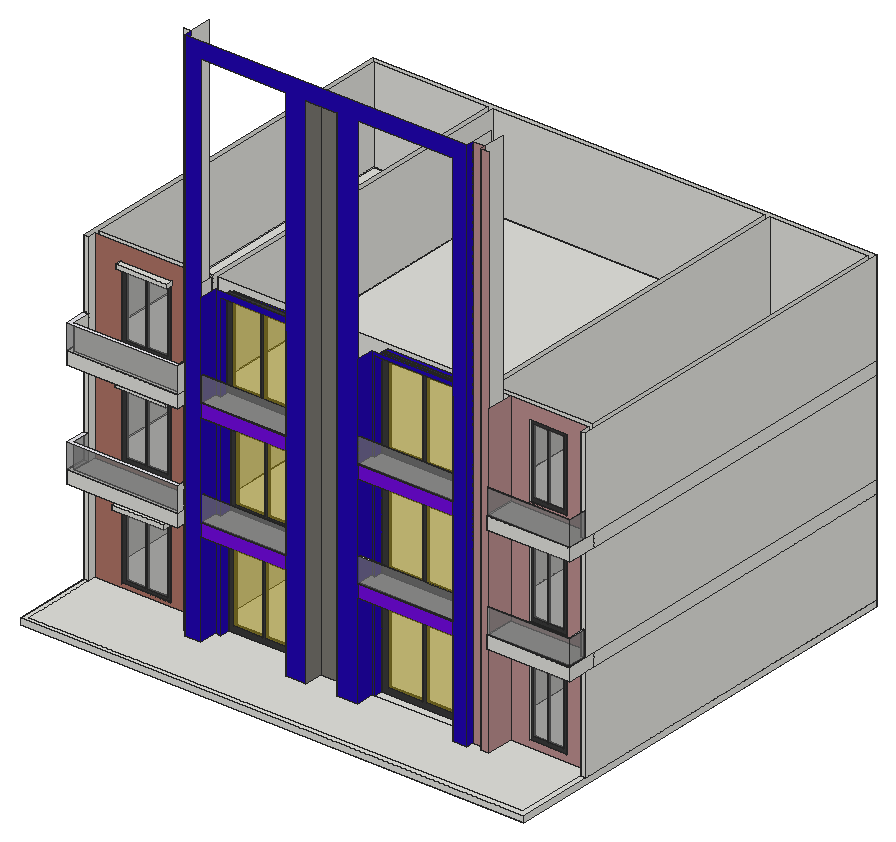
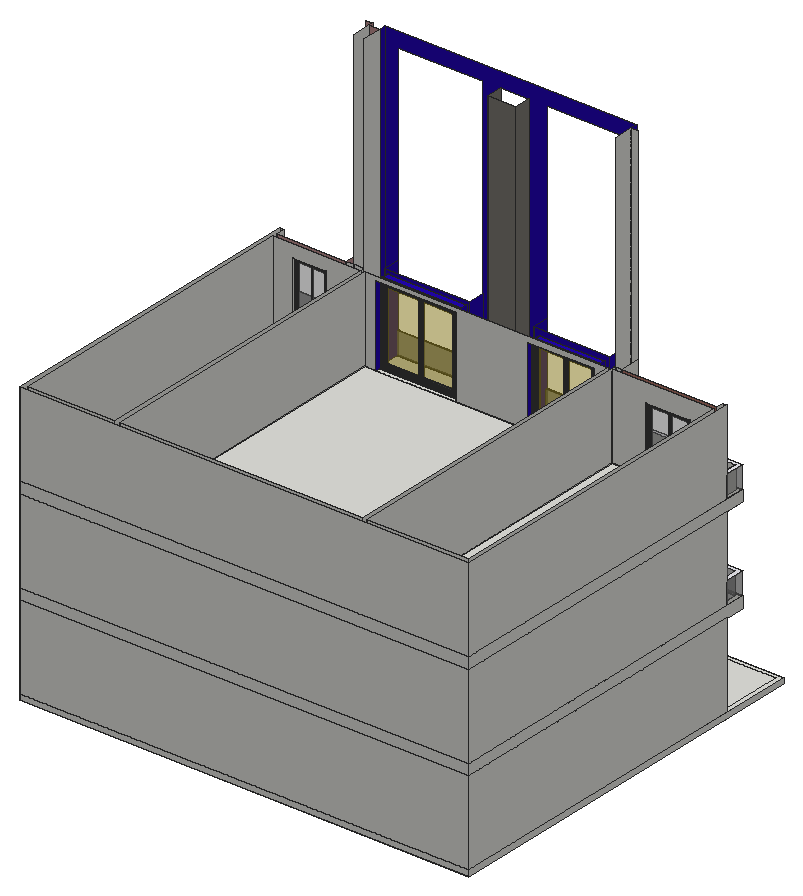
# SketchUp Ruby script. Lengths in inches.
U = 1.inch
M = Sketchup.active_model
def pt(a) = Geom::Point3d.new(a.map { |v| v * U })
def face(e, loops, mat)
  f = e.add_face(loops[0].map { |a| pt(a) })
  loops[1..].each { |l| e.add_face(l.map { |a| pt(a) }).erase! }
  f.material = f.back_material = mat if mat
  f
end
# faces: each face lists its corners as indices into pts; further lists are holes
def faces(e, pts, list, mat = nil) = list.each { |f| face(e, (f[0].is_a?(Array) ? f : [f]).map { |l| l.map { |i| pts[i] } }, mat) }
# xy, xz, yz: faces in a plane at the given z, y or x. An outline is a flat list of corners, or four numbers for a rectangle; further outlines are holes
def ring(l) = l.size == 4 ? [[l[0], l[1]], [l[2], l[1]], [l[2], l[3]], [l[0], l[3]]] : l.each_slice(2).to_a
def flat(e, list, mat, &to3) = list.each { |f| face(e, (f[0].is_a?(Array) ? f : [f]).map { |l| ring(l).map { |u, v| to3.(u, v) } }, mat) }
def xy(e, z, list, mat = nil) = flat(e, list, mat) { |x, y| [x, y, z] }
def xz(e, y, list, mat = nil) = flat(e, list, mat) { |x, z| [x, y, z] }
def yz(e, x, list, mat = nil) = flat(e, list, mat) { |y, z| [x, y, z] }
def lines(e, pts, list) = list.each { |a, b| e.add_line(pt(pts[a]), pt(pts[b])) }
# prism: a flat outline (further loops are holes) pulled along v
def prism(e, loops, v, mat = nil)
  f = face(e, loops, mat); d = Geom::Vector3d.new(v.map { |x| x * U })
  f.pushpull(f.normal.samedirection?(d) ? d.length : -d.length)
end
def box(e, o, s, mat = nil) = prism(e, [[o, [o[0] + s[0], o[1], o[2]], [o[0] + s[0], o[1] + s[1], o[2]], [o[0], o[1] + s[1], o[2]]]], [0, 0, s[2]], mat)
def at(x, y, z, deg = 0) = Geom::Transformation.translation(pt([x, y, z])) * Geom::Transformation.rotation(ORIGIN, Z_AXIS, deg.degrees)
def axes(o, x, y, z) = Geom::Transformation.new([*x, 0, *y, 0, *z, 0, *pt(o).to_a, 1])
def part(name) = M.definitions.add(name)
# library, detail: a bought-in or finely detailed component or shape, given as its bounding box
def library(name, o, s) = part(name).tap { |d| box(d.entities, o, s) }
def detail(e, o, s) = box(e.add_group.entities, o, s)
def put(e, d, t, mat = nil) = e.add_instance(d, t).tap { |i| i.material = mat if mat }
def group(e, t, mat = nil) = e.add_group.tap { |g| g.transformation = t; g.material = mat if mat }.entities
root = M.entities
M.materials.add("[0119_RosyBrown]").color = [188, 143, 143]
M.materials.add("[Brick Colored Blue]").color = [34, 5, 180]
M.materials.add("[Brick Colored Blue]1").color = [115, 11, 225]
M.materials.add("[Color M07]").color = [58, 58, 58]
M.materials.add("[Metal Silver]").color = [234, 233, 238]
M.materials.add("[Rough Square Concrete Block]").color = [123, 120, 113]
M.materials.add("[Stone Flagstone Ashlar]").color = [175, 116, 102]
M.materials.add("[Translucent Glass Blue]").color = [202, 178, 24]
M.materials["[Translucent Glass Blue]"].alpha = 0.5
M.materials.add("[Translucent Glass Gray]").color = [128, 128, 128]
M.materials["[Translucent Glass Gray]"].alpha = 0.5
c1 = part("Group\#2")
xy(c1.entities,0,[[0,0,124.375,6.5]],"[Color M07]")
xy(c1.entities,9.35,[[9.35,0,58.13,6.5],[62.66,0,115.02,6.5]],"[Color M07]")
xy(c1.entities,131.58,[[9.35,0,58.13,6.5],[62.66,0,115.02,6.5]],"[Color M07]")
xy(c1.entities,140.9375,[[0,0,124.375,6.5]],"[Color M07]")
xz(c1.entities,0,[[[0,0,124.375,140.9375],[62.66,9.35,115.02,131.58],[9.35,9.35,58.13,131.58]]],"[Color M07]")
xz(c1.entities,0,[[9.35,9.35,58.13,131.58],[62.66,9.35,115.02,131.58]],"[Translucent Glass Blue]")
xz(c1.entities,6.5,[[[0,0,124.375,140.9375],[62.66,9.35,115.02,131.58],[9.35,9.35,58.13,131.58]]],"[Color M07]")
yz(c1.entities,0,[[0,0,6.5,140.9375]],"[Color M07]")
yz(c1.entities,9.35,[[0,9.35,6.5,131.58]],"[Color M07]")
yz(c1.entities,58.13,[[0,9.35,6.5,131.58]],"[Color M07]")
yz(c1.entities,62.66,[[0,9.35,6.5,131.58]],"[Color M07]")
yz(c1.entities,115.02,[[0,9.35,6.5,131.58]],"[Color M07]")
yz(c1.entities,124.375,[[0,0,6.5,140.9375]],"[Color M07]")
c2 = part("Group\#1")
xy(c2.entities,0,[[0,0,103.0625,5.375]],"[Color M07]")
xy(c2.entities,8.61,[[8.61,0,48.54,5.375],[51.97,0,94.45,5.375]],"[Color M07]")
xy(c2.entities,158.15,[[8.61,0,48.54,5.375],[51.97,0,94.45,5.375]],"[Color M07]")
xy(c2.entities,166.76,[[0,0,103.0625,5.375]],"[Color M07]")
xz(c2.entities,0,[[[0,0,103.0625,166.76],[51.97,8.61,94.45,158.15],[8.61,8.61,48.54,158.15]]],"[Color M07]")
xz(c2.entities,0,[[8.61,8.61,48.54,158.15],[51.97,8.61,94.45,158.15]],"[Translucent Glass Gray]")
xz(c2.entities,5.375,[[[0,0,103.0625,166.76],[51.97,8.61,94.45,158.15],[8.61,8.61,48.54,158.15]]],"[Color M07]")
yz(c2.entities,0,[[0,0,5.375,166.76]],"[Color M07]")
yz(c2.entities,8.61,[[0,8.61,5.375,158.15]],"[Color M07]")
yz(c2.entities,48.54,[[0,8.61,5.375,158.15]],"[Color M07]")
yz(c2.entities,51.97,[[0,8.61,5.375,158.15]],"[Color M07]")
yz(c2.entities,94.45,[[0,8.61,5.375,158.15]],"[Color M07]")
yz(c2.entities,103.0625,[[0,0,5.375,166.76]],"[Color M07]")
xy(root,0,[[0,0,960,840]])
xy(root,12,[[0,0,960,0,960,147.0625,951,147.0625,951,9,9,9,9,151.625,0,151.625],[9,9,951,9,951,166.4375,801.6875,166.4375,801.6875,115.3125,786.375,115.3125,786.375,124.625,763.625,124.625,763.625,110.3125,736.375,110.3125,736.375,145,554.39,145,554.39,110.3125,515.65,110.3125,515.65,145,456.7,145,456.7,110.3125,417.96,110.3125,417.96,145,405.4,145,405.4,175.4375,265.83,175.4375,265.83,145,255.8125,145,255.8125,110.3125,226.3125,110.3125,226.3125,124.375,212.1875,124.375,212.1875,166.4375,9,166.4375],[[226.3125,110.3125,226.3125,166.4375,9,166.4375,9,151.625,0,151.625,0,840,960,840,960,147.0625,951,147.0625,951,166.4375,763.625,166.4375,763.625,110.3125,736.375,110.3125,736.375,145,730.3125,145,730.3125,175.4375,754.625,175.4375,754.625,831,235.3125,831,235.3125,175.4375,265.83,175.4375,265.83,145,255.8125,145,255.8125,110.3125],[9,175.4375,226.3125,831],[763.625,175.4375,951,831]],[417.96,110.3125,417.96,145,405.4,145,405.4,175.4375,560.75,175.4375,560.75,145,554.39,145,554.39,110.3125,515.65,110.3125,515.65,145,456.7,145,456.7,110.3125],[786.375,115.3125,801.6875,166.4375],
  [212.1875,124.375,226.3125,166.4375],[763.625,124.625,786.375,166.4375],[560.75,145,730.3125,175.4375],[9,175.4375,226.3125,831],[235.3125,175.4375,754.625,831],
  [763.625,175.4375,951,831]])
xy(root,19.77,[[59.43,166.4375,154.62,175.4375]])
xy(root,24.53,[[838.25,166.4375,907.94,175.4375]])
xy(root,152.51,[[57.84,146.25,57.84,166.4375,59.43,166.4375,59.43,175.4375,154.62,175.4375,154.62,166.4375,155.9,166.4375,155.9,146.25]])
xy(root,162.04,[[57.84,146.25,155.9,166.4375]])
xy(root,164.9,[[838.25,166.4375,907.94,175.4375]])
xy(root,178.5,[[265.83,145,405.4,175.4375]],"[Brick Colored Blue]")
xy(root,184.85,[[560.75,145,730.3125,175.4375]],"[Brick Colored Blue]")
xy(root,192,[[0,110.3125,9,151.625],[9,110.3125,212.1875,166.4375],[255.8125,110.3125,417.96,145],[554.39,110.3125,736.375,145],[801.6875,110.3125,801.6875,166.4375,951,166.4375,951,147.0625,960,147.0625,960,110.3125]])
xy(root,210,[[9,175.4375,226.3125,831],[235.3125,175.4375,754.625,831]])
xy(root,213,[[763.625,175.4375,951,831]])
xy(root,216,[[0,110.3125,0,151.625,9,151.625,9,117.34,210.0625,117.34,210.0625,124.375,212.1875,124.375,212.1875,110.3125],[255.8125,110.3125,417.96,111.6875],[554.39,110.3125,736.375,111.6875],[801.6875,110.3125,960,110.3125,960,147.0625,959.125,147.0625,959.125,110.8125,801.6875,110.8125],[801.6875,110.8125,802.5,115.3125],
  [802.5,110.8125,802.5,113,956.625,113,956.625,147.0625,959.125,147.0625,959.125,110.8125],[255.8125,111.6875,417.96,113.6875],[554.39,111.6875,736.375,113.6875],[802.5,113,956.625,113,956.625,147.0625,951,147.0625,951,166.4375,801.6875,166.4375,801.6875,115.3125,802.5,115.3125],[255.8125,113.6875,417.96,113.6875,417.96,145,405.4,145,405.4,175.4375,265.83,175.4375,265.83,145,255.8125,145],
  [554.39,113.6875,736.375,113.6875,736.375,145,730.3125,145,730.3125,175.4375,560.75,175.4375,560.75,145,554.39,145],[9,117.34,210.0625,117.34,210.0625,124.375,212.1875,124.375,212.1875,166.4375,9,166.4375],[9,175.4375,226.3125,831],[235.3125,175.4375,754.625,831],[763.625,175.4375,951,831]])
xy(root,226.89,[[59.43,166.4375,154.62,175.4375]])
xy(root,227.09,[[838.25,166.4375,907.94,175.4375]])
xy(root,264,[[0,110.3125,212.1875,110.3125,212.1875,124.375,210.0625,124.375,210.0625,117.34,9,117.34,9,151.625,0,151.625],[802.5,110.8125,959.125,110.8125,959.125,147.0625,956.625,147.0625,956.625,113,802.5,113],[255.8125,111.6875,417.96,113.6875],[554.39,111.6875,736.375,113.6875]],"[Metal Silver]")
xy(root,359.63,[[57.84,152.125,57.84,166.4375,59.43,166.4375,59.43,175.4375,154.62,175.4375,154.62,166.4375,155.9,166.4375,155.9,152.125]])
xy(root,367.47,[[838.25,166.4375,907.94,175.4375]])
xy(root,368.04,[[57.84,152.125,155.9,166.4375]])
xy(root,382.81,[[265.83,145,405.4,175.4375]],"[Brick Colored Blue]")
xy(root,387.91,[[560.75,145,730.3125,175.4375]])
xy(root,396,[[0,110.3125,9,151.625],[9,110.3125,212.1875,166.4375],[255.8125,110.3125,417.96,145],[554.39,110.3125,736.375,145],[801.6875,110.3125,801.6875,166.4375,951,166.4375,951,147.0625,960,147.0625,960,110.3125]])
xy(root,409.875,[[763.625,175.4375,951,831]])
xy(root,414,[[9,175.4375,226.3125,831],[235.3125,175.4375,754.625,831]])
xy(root,420,[[0,110.3125,0,151.625,9,151.625,9,117.34,208.125,117.34,208.125,124.375,212.1875,124.375,212.1875,110.3125],[255.8125,110.3125,417.96,111.8125],[554.39,110.3125,736.375,111.8125],[801.6875,110.3125,960,110.3125,960,147.0625,959.6875,147.0625,959.6875,110.8125,801.6875,110.8125],[801.6875,110.8125,802.125,115.3125],
  [802.125,110.8125,802.125,111.5625,958.9375,111.5625,958.9375,147.0625,959.6875,147.0625,959.6875,110.8125],[802.125,111.5625,958.9375,111.5625,958.9375,147.0625,951,147.0625,951,166.4375,801.6875,166.4375,801.6875,115.3125,802.125,115.3125],[255.8125,111.8125,417.96,113.8125],[554.39,111.8125,736.375,113.8125],[255.8125,113.8125,417.96,113.8125,417.96,145,405.4,145,405.4,175.4375,265.83,175.4375,265.83,145,255.8125,145],
  [554.39,113.8125,736.375,113.8125,736.375,145,730.3125,145,730.3125,175.4375,560.75,175.4375,560.75,145,554.39,145],[9,117.34,208.125,117.34,208.125,124.375,212.1875,124.375,212.1875,166.4375,9,166.4375],[9,175.4375,226.3125,831],[235.3125,175.4375,754.625,831],[763.625,175.4375,951,831]])
xy(root,428.14,[[59.43,166.4375,154.62,175.4375]])
xy(root,432.47,[[838.25,166.4375,907.94,175.4375]])
xy(root,468,[[802.125,110.8125,959.6875,110.8125,959.6875,147.0625,958.9375,147.0625,958.9375,111.5625,802.125,111.5625]])
xy(root,468,[[255.8125,111.8125,417.96,113.8125],[554.39,111.8125,736.375,113.8125]],"[Metal Silver]")
xy(root,468.3125,[[0,110.3125,212.1875,110.3125,212.1875,124.375,208.125,124.375,208.125,117.34,9,117.34,9,151.625,0,151.625]],"[Metal Silver]")
xy(root,560.88,[[57.84,154.25,57.84,166.4375,59.43,166.4375,59.43,175.4375,154.62,175.4375,154.62,166.4375,155.9,166.4375,155.9,154.25]])
xy(root,568.66,[[57.84,154.25,155.9,166.4375]])
xy(root,572.84,[[838.25,166.4375,907.94,175.4375]])
xy(root,587.81,[[265.83,145,405.4,175.4375]],"[Brick Colored Blue]")
xy(root,592.22,[[560.75,145,730.3125,175.4375]],"[Brick Colored Blue]")
xz(root,0,[[0,0,960,12]])
xz(root,110.3125,[[0,192,212.1875,216],[801.6875,192,960,216],[0,396,212.1875,420],[801.6875,396,960,420]])
xz(root,110.3125,[[226.3125,12,255.8125,12,255.8125,1008,417.96,1008,417.96,12,456.7,12,456.7,1008,515.65,1008,515.65,12,554.39,12,554.39,1008,736.375,1008,736.375,12,763.625,12,763.625,1039.1875,226.3125,1039.1875]],"[Brick Colored Blue]")
xz(root,110.3125,[[255.8125,192,417.96,216],[554.39,192,736.375,216],[255.8125,396,417.96,420],[554.39,396,736.375,420]],"[Brick Colored Blue]1")
xz(root,110.3125,[[0,216,212.1875,264],[0,420,212.1875,468.3125]],"[Translucent Glass Gray]")
xz(root,110.8125,[[802.5,216,959.125,264],[802.125,420,959.6875,468]],"[Translucent Glass Gray]")
xz(root,111.5625,[[802.125,420,958.9375,468]],"[Translucent Glass Gray]")
xz(root,111.6875,[[255.8125,216,417.96,264],[554.39,216,736.375,264]],"[Translucent Glass Gray]")
xz(root,111.8125,[[255.8125,420,417.96,468],[554.39,420,736.375,468]],"[Translucent Glass Gray]")
xz(root,113,[[802.5,216,956.625,264]],"[Translucent Glass Gray]")
xz(root,113.6875,[[255.8125,216,417.96,264],[554.39,216,736.375,264]],"[Translucent Glass Gray]")
xz(root,113.8125,[[255.8125,420,417.96,468],[554.39,420,736.375,468]],"[Translucent Glass Gray]")
xz(root,115.3125,[[786.375,12,801.6875,1039.1875]],"[0119_RosyBrown]")
xz(root,117.34,[[9,420,208.125,468.3125]])
xz(root,117.34,[[9,216,210.0625,264]],"[Translucent Glass Gray]")
xz(root,124.375,[[212.1875,12,226.3125,1039.1875],[210.0625,216,212.1875,264],[208.125,420,212.1875,468.3125],[226.3125,420,229.5,600]])
xz(root,124.625,[[763.625,12,786.375,1039.1875]],"[0119_RosyBrown]")
xz(root,145,[[255.8125,12,265.83,12,265.83,178.5,405.4,178.5,405.4,12,417.96,12,417.96,192,255.8125,192],[554.39,12,560.75,12,560.75,184.85,730.3125,184.85,730.3125,12,736.375,12,736.375,192,554.39,192],[255.8125,216,265.83,216,265.83,382.81,405.4,382.81,405.4,216,417.96,216,417.96,396,255.8125,396],[554.39,216,560.75,216,560.75,387.91,730.3125,387.91,730.3125,216,736.375,216,736.375,396,554.39,396],[255.8125,420,265.83,420,265.83,587.81,405.4,587.81,405.4,420,417.96,420,417.96,600,255.8125,600],
  [554.39,420,560.75,420,560.75,592.22,730.3125,592.22,730.3125,420,736.375,420,736.375,600,554.39,600]],"[Brick Colored Blue]")
xz(root,145,[[456.7,12,515.65,1008]],"[Rough Square Concrete Block]")
xz(root,146.25,[[57.84,152.51,155.9,162.04]])
xz(root,147.0625,[[951,12,960,192],[951,216,956.625,216,956.625,264,959.125,264,959.125,216,960,216,960,396,951,396],[956.625,216,959.125,264],[951,420,958.9375,420,958.9375,468,959.6875,468,959.6875,420,960,420,960,600,951,600],[958.9375,420,959.6875,468]])
xz(root,151.625,[[2.39,-3.36,6.71,0.95],[2.39,5.08,6.71,9.39],[0,12,9,192],[2.38,209.32,6.44,213.38],[0,216,9,264],
  [0,264,9,396],[2.1,413.18,6.41,417.5],[0,420,9,468],[0,468,9,468.3125],[0,468.3125,9,600]])
xz(root,152.125,[[57.84,359.63,155.9,368.04]])
xz(root,154.25,[[57.84,560.88,155.9,568.66]])
xz(root,166.4375,[[212.1875,12,226.3125,192],[763.625,12,786.375,192],[786.375,12,801.6875,192],[217.1875,192,226.3125,216],[763.625,192,786.375,216],
  [786.375,192,801.6875,216],[212.1875,216,226.3125,396],[763.625,216,786.375,396],[786.375,216,801.6875,396],[217.1875,396,226.3125,420],
  [763.625,396,786.375,420],[786.375,396,801.6875,420],[212.1875,420,226.3125,600],[226.3125,420,229.5,600],[763.625,420,786.375,600],
  [786.375,420,801.6875,600]])
xz(root,166.4375,[[[801.6875,12,951,192],[838.25,24.53,907.94,164.9]],[[801.6875,216,951,396],[838.25,227.09,907.94,367.47]],[[801.6875,420,951,600],[838.25,432.47,907.94,572.84]]],"[0119_RosyBrown]")
xz(root,166.4375,[[[9,12,212.1875,192],[59.43,19.77,59.43,152.51,57.84,152.51,57.84,162.04,155.9,162.04,155.9,152.51,154.62,152.51,154.62,19.77]],[[9,216,212.1875,396],[59.43,226.89,59.43,359.63,57.84,359.63,57.84,368.04,155.9,368.04,155.9,359.63,154.62,359.63,154.62,226.89]],[[9,420,212.1875,600],[59.43,428.14,59.43,560.88,57.84,560.88,57.84,568.66,155.9,568.66,155.9,560.88,154.62,560.88,154.62,428.14]]],"[Stone Flagstone Ashlar]")
xz(root,175.4375,[[[9,12,226.3125,192],[59.43,19.77,154.62,152.51]],[235.3125,12,235.3125,192,754.625,192,754.625,12,730.3125,12,730.3125,184.85,560.75,184.85,560.75,12,405.4,12,405.4,178.5,265.83,178.5,265.83,12],[[763.625,12,951,192],[838.25,24.53,907.94,164.9]],[9,192,226.3125,210],[235.3125,192,754.625,210],
  [763.625,192,951,213],[9,210,226.3125,216],[235.3125,210,265.83,216],[265.83,210,405.4,216],[405.4,210,560.75,216],
  [560.75,210,730.3125,216],[730.3125,210,754.625,216],[763.625,213,951,216],[[9,216,226.3125,396],[59.43,226.89,154.62,359.63]],[235.3125,216,235.3125,396,754.625,396,754.625,216,730.3125,216,730.3125,387.91,560.75,387.91,560.75,216,405.4,216,405.4,382.81,265.83,382.81,265.83,216],
  [[763.625,216,951,396],[838.25,227.09,907.94,367.47]],[9,396,226.3125,414],[235.3125,396,754.625,414],[763.625,396,951,409.875],[763.625,409.875,951,420],
  [9,414,226.3125,420],[235.3125,414,265.83,420],[265.83,414,405.4,420],[405.4,414,560.75,420],[560.75,414,730.3125,420],
  [730.3125,414,754.625,420],[[9,420,226.3125,600],[59.43,428.14,154.62,560.88]],[235.3125,420,235.3125,600,754.625,600,754.625,420,730.3125,420,730.3125,592.22,560.75,592.22,560.75,420,405.4,420,405.4,587.81,265.83,587.81,265.83,420],[[763.625,420,951,600],[838.25,432.47,907.94,572.84]]])
xz(root,831,[[9,12,226.3125,192],[235.3125,12,754.625,192],[763.625,12,951,192],[9,192,226.3125,210],[235.3125,192,754.625,210],
  [763.625,192,951,213],[9,210,226.3125,216],[235.3125,210,754.625,216],[763.625,213,951,216],[9,216,226.3125,396],
  [235.3125,216,754.625,396],[763.625,216,951,396],[9,396,226.3125,414],[235.3125,396,754.625,414],[763.625,396,951,409.875],
  [763.625,409.875,951,420],[9,414,226.3125,420],[235.3125,414,754.625,420],[9,420,226.3125,600],[235.3125,420,754.625,600],
  [763.625,420,951,600]])
xz(root,840,[[0,0,960,12],[0,12,960,192],[0,192,960,216],[0,216,960,396],[0,396,960,420],
  [0,420,960,600]])
yz(root,0,[[0,0,840,12],[151.625,12,840,192],[110.3125,192,840,216],[151.625,216,840,396],[110.3125,396,840,420],
  [151.625,420,840,600]])
yz(root,0,[[110.3125,216,151.625,264],[110.3125,420,151.625,468.3125]],"[Translucent Glass Gray]")
yz(root,9,[[151.625,12,166.4375,192],[175.4375,12,831,192],[175.4375,192,831,210],[175.4375,210,200.26,216],[200.26,210,214.57,216],
  [214.57,210,831,216],[151.625,216,166.4375,396],[175.4375,216,831,396],[175.4375,396,831,414],[175.4375,414,236.35,420],
  [236.35,414,248.35,420],[248.35,414,831,420],[117.34,420,151.625,468.3125],[151.625,420,166.4375,600],[175.4375,420,831,600]])
yz(root,9,[[117.34,216,151.625,264]],"[Translucent Glass Gray]")
yz(root,57.84,[[146.25,152.51,166.4375,162.04],[152.125,359.63,166.4375,368.04],[154.25,560.88,166.4375,568.66]])
yz(root,59.43,[[166.4375,19.77,175.4375,152.51],[166.4375,226.89,175.4375,359.63],[166.4375,428.14,175.4375,560.88]])
yz(root,154.62,[[166.4375,19.77,175.4375,152.51],[166.4375,226.89,175.4375,359.63],[166.4375,428.14,175.4375,560.88]])
yz(root,155.9,[[146.25,152.51,166.4375,162.04],[152.125,359.63,166.4375,368.04],[154.25,560.88,166.4375,568.66]])
yz(root,208.125,[[117.34,420,124.375,468.3125]])
yz(root,210.0625,[[117.34,216,124.375,264]])
yz(root,212.1875,[[124.375,12,166.4375,192],[110.3125,192,124.375,216],[110.3125,216,124.375,264],[124.375,216,166.4375,396],[110.3125,396,124.375,420],
  [110.3125,420,124.375,468.3125],[124.375,420,166.4375,600]])
yz(root,226.3125,[[124.375,12,166.4375,1039.1875],[175.4375,12,831,192],[175.4375,192,831,210],[175.4375,210,831,216],[166.4375,216,175.4375,396],
  [175.4375,216,831,396],[166.4375,396,175.4375,420],[175.4375,396,831,414],[175.4375,414,831,420],[166.4375,420,175.4375,600],
  [175.4375,420,831,600]])
yz(root,226.3125,[[110.3125,12,124.375,1039.1875]],"[Brick Colored Blue]")
yz(root,229.5,[[124.375,420,166.4375,600]])
yz(root,235.3125,[[175.4375,12,831,192],[175.4375,192,831,210],[175.4375,210,196.77,216],[196.77,210,256.71,216],[256.71,210,831,216],
  [175.4375,216,831,396],[175.4375,396,831,414],[175.4375,414,216.11,420],[216.11,414,230.67,420],[230.67,414,831,420],
  [175.4375,420,831,600]])
yz(root,255.8125,[[111.6875,216,113.6875,264],[111.8125,420,113.8125,468]])
yz(root,255.8125,[[110.3125,12,145,192],[110.3125,216,111.6875,216,111.6875,264,113.6875,264,113.6875,216,145,216,145,396,110.3125,396],[110.3125,420,111.8125,420,111.8125,468,113.8125,468,113.8125,420,145,420,145,600,110.3125,600]],"[Brick Colored Blue]")
yz(root,265.83,[[145,12,175.4375,178.5],[145,216,175.4375,382.81],[145,420,175.4375,587.81]],"[Brick Colored Blue]")
yz(root,405.4,[[145,12,175.4375,178.5],[145,216,175.4375,382.81],[145,420,175.4375,587.81]],"[Brick Colored Blue]")
yz(root,417.96,[[111.6875,216,113.6875,264],[111.8125,420,113.8125,468]])
yz(root,417.96,[[110.3125,12,145,192],[110.3125,216,110.3125,396,145,396,145,216,113.6875,216,113.6875,264,111.6875,264,111.6875,216],[110.3125,420,110.3125,600,145,600,145,420,113.8125,420,113.8125,468,111.8125,468,111.8125,420]],"[Brick Colored Blue]")
yz(root,456.7,[[110.3125,12,145,1008]],"[Rough Square Concrete Block]")
yz(root,515.65,[[110.3125,12,145,1008]],"[Rough Square Concrete Block]")
yz(root,554.39,[[111.6875,216,113.6875,264],[111.8125,420,113.8125,468]])
yz(root,554.39,[[110.3125,12,145,192],[110.3125,216,111.6875,216,111.6875,264,113.6875,264,113.6875,216,145,216,145,396,110.3125,396],[110.3125,420,111.8125,420,111.8125,468,113.8125,468,113.8125,420,145,420,145,600,110.3125,600]],"[Brick Colored Blue]")
yz(root,560.75,[[145,12,175.4375,184.85],[145,216,175.4375,387.91],[145,420,175.4375,592.22]],"[Brick Colored Blue]")
yz(root,730.3125,[[145,12,175.4375,184.85],[145,216,175.4375,387.91],[145,420,175.4375,592.22]],"[Brick Colored Blue]")
yz(root,736.375,[[111.6875,216,113.6875,264],[111.8125,420,113.8125,468]])
yz(root,736.375,[[110.3125,12,145,192],[110.3125,216,110.3125,396,145,396,145,216,113.6875,216,113.6875,264,111.6875,264,111.6875,216],[110.3125,420,110.3125,600,145,600,145,420,113.8125,420,113.8125,468,111.8125,468,111.8125,420]],"[Brick Colored Blue]")
yz(root,754.625,[[175.4375,12,831,192],[175.4375,192,831,210],[175.4375,210,831,216],[175.4375,216,831,396],[175.4375,396,831,414],
  [175.4375,414,831,420],[175.4375,420,831,600]])
yz(root,763.625,[[124.625,12,166.4375,1039.1875],[175.4375,12,831,192],[175.4375,192,831,213],[175.4375,213,185.38,216],[185.38,213,199.57,216],
  [199.57,213,831,216],[166.4375,216,175.4375,396],[175.4375,216,831,396],[166.4375,396,175.4375,420],[175.4375,396,831,409.875],
  [175.4375,409.875,195.28,420],[195.28,409.875,199.57,420],[199.57,409.875,831,420],[166.4375,420,175.4375,600],[175.4375,420,831,600]])
yz(root,763.625,[[110.3125,12,124.625,1039.1875]],"[Brick Colored Blue]")
yz(root,786.375,[[124.625,12,166.4375,1039.1875]])
yz(root,786.375,[[115.3125,12,124.625,1039.1875]],"[0119_RosyBrown]")
yz(root,801.6875,[[110.3125,192,115.3125,216],[115.3125,192,166.4375,216],[110.3125,396,115.3125,420],[115.3125,396,166.4375,420]])
yz(root,801.6875,[[115.3125,12,166.4375,192],[115.3125,216,166.4375,396],[115.3125,420,166.4375,600]],"[0119_RosyBrown]")
yz(root,802.125,[[110.8125,420,111.5625,468]])
yz(root,802.5,[[110.8125,216,113,264]])
yz(root,838.25,[[166.4375,24.53,175.4375,164.9],[166.4375,227.09,175.4375,367.47],[166.4375,432.47,175.4375,572.84]])
yz(root,907.94,[[166.4375,24.53,175.4375,164.9],[166.4375,227.09,175.4375,367.47],[166.4375,432.47,175.4375,572.84]])
yz(root,951,[[147.0625,12,166.4375,192],[175.4375,12,831,192],[175.4375,192,831,213],[175.4375,213,831,216],[147.0625,216,166.4375,396],
  [175.4375,216,831,396],[175.4375,396,831,409.875],[175.4375,409.875,831,420],[147.0625,420,166.4375,600],[175.4375,420,831,600]])
yz(root,956.625,[[113,216,147.0625,264]],"[Translucent Glass Gray]")
yz(root,958.9375,[[111.5625,420,147.0625,468]],"[Translucent Glass Gray]")
yz(root,959.125,[[110.8125,216,147.0625,264]],"[Translucent Glass Gray]")
yz(root,959.6875,[[110.8125,420,147.0625,468]],"[Translucent Glass Gray]")
yz(root,960,[[0,0,840,12],[147.0625,12,840,192],[110.3125,192,166.4375,216],[166.4375,192,840,216],[147.0625,216,840,396],
  [110.3125,396,166.4375,420],[166.4375,396,840,420],[147.0625,420,840,600]])
p = [[515.65,145,12],[515.65,145,3.875],[217.1875,166.4375,396],[217.1875,124.375,396],[217.1875,166.4375,420],[217.1875,124.375,420],
  [217.1875,166.4375,216],[217.1875,124.375,216],[217.1875,166.4375,192],[217.1875,124.375,192]]
lines(root,p,[[0,1],[2,3],[4,5],[6,7],[8,9]])
put(root,c1,axes([560.75,160.22,12],[1.36332,0,0],[0,1,0],[0,0,1.22243]))
put(root,c1,axes([265.83,163.94,12],[1.12211,0,0],[0,1,0],[0,0,1.18134]))
put(root,c2,axes([59.43,168.6875,17.52],[0.92359,0,0],[0,0.65,0],[0,0,0.81192]))
put(root,c2,axes([838.25,168.1875,24.53],[0.67617,0,0],[0,0.325,0],[0,0,0.84179]))
put(root,c1,axes([265.83,168.9375,216],[1.12211,0,0],[0,1,0],[0,0,1.20218]))
put(root,c1,axes([560.75,160.22,216],[1.36332,0,0],[0,1,0],[0,0,1.22243]))
put(root,c2,axes([59.43,168.6875,226.89],[0.92359,0,0],[0,0.65,0],[0,0,0.796]))
put(root,c2,axes([838.25,168.1875,227.65],[0.67617,0,0],[0,0.325,0],[0,0,0.84179]))
put(root,c1,axes([560.75,160.22,420],[1.36332,0,0],[0,1,0],[0,0,1.22243]))
put(root,c1,axes([265.83,160.22,421.125],[1.12211,0,0],[0,1,0],[0,0,1.20218]),"[Brick Colored Blue]")
put(root,c2,axes([59.43,168.6875,428.14],[0.92359,0,0],[0,0.65,0],[0,0,0.796]))
put(root,c2,axes([838.25,168.1875,432.47],[0.67617,0,0],[0,0.325,0],[0,0,0.84179]))
